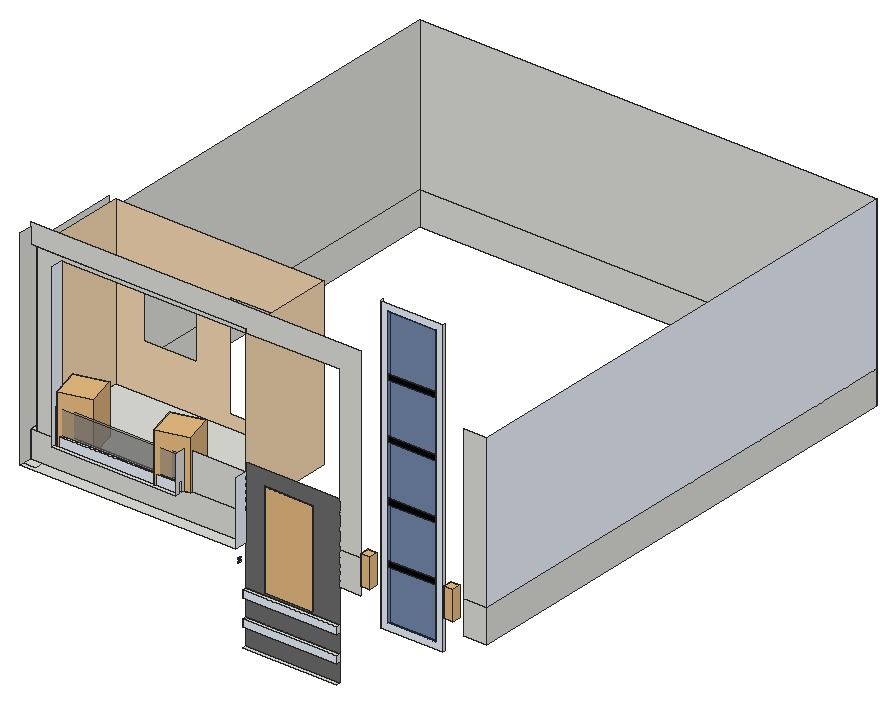
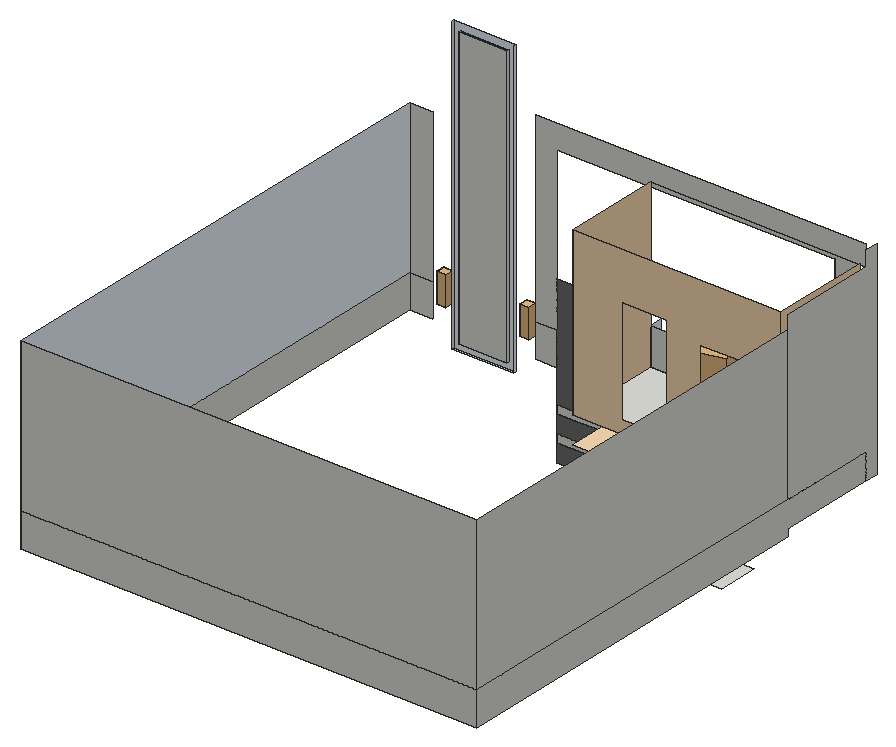
# SketchUp Ruby script. Lengths in inches.
U = 1.inch
M = Sketchup.active_model
def pt(a) = Geom::Point3d.new(a.map { |v| v * U })
def face(e, loops, mat)
  f = e.add_face(loops[0].map { |a| pt(a) })
  loops[1..].each { |l| e.add_face(l.map { |a| pt(a) }).erase! }
  f.material = f.back_material = mat if mat
  f
end
# faces: each face lists its corners as indices into pts; further lists are holes
def faces(e, pts, list, mat = nil) = list.each { |f| face(e, (f[0].is_a?(Array) ? f : [f]).map { |l| l.map { |i| pts[i] } }, mat) }
# xy, xz, yz: faces in a plane at the given z, y or x. An outline is a flat list of corners, or four numbers for a rectangle; further outlines are holes
def ring(l) = l.size == 4 ? [[l[0], l[1]], [l[2], l[1]], [l[2], l[3]], [l[0], l[3]]] : l.each_slice(2).to_a
def flat(e, list, mat, &to3) = list.each { |f| face(e, (f[0].is_a?(Array) ? f : [f]).map { |l| ring(l).map { |u, v| to3.(u, v) } }, mat) }
def xy(e, z, list, mat = nil) = flat(e, list, mat) { |x, y| [x, y, z] }
def xz(e, y, list, mat = nil) = flat(e, list, mat) { |x, z| [x, y, z] }
def yz(e, x, list, mat = nil) = flat(e, list, mat) { |y, z| [x, y, z] }
def lines(e, pts, list) = list.each { |a, b| e.add_line(pt(pts[a]), pt(pts[b])) }
# prism: a flat outline (further loops are holes) pulled along v
def prism(e, loops, v, mat = nil)
  f = face(e, loops, mat); d = Geom::Vector3d.new(v.map { |x| x * U })
  f.pushpull(f.normal.samedirection?(d) ? d.length : -d.length)
end
def box(e, o, s, mat = nil) = prism(e, [[o, [o[0] + s[0], o[1], o[2]], [o[0] + s[0], o[1] + s[1], o[2]], [o[0], o[1] + s[1], o[2]]]], [0, 0, s[2]], mat)
def at(x, y, z, deg = 0) = Geom::Transformation.translation(pt([x, y, z])) * Geom::Transformation.rotation(ORIGIN, Z_AXIS, deg.degrees)
def axes(o, x, y, z) = Geom::Transformation.new([*x, 0, *y, 0, *z, 0, *pt(o).to_a, 1])
def part(name) = M.definitions.add(name)
# library, detail: a bought-in or finely detailed component or shape, given as its bounding box
def library(name, o, s) = part(name).tap { |d| box(d.entities, o, s) }
def detail(e, o, s) = box(e.add_group.entities, o, s)
def put(e, d, t, mat = nil) = e.add_instance(d, t).tap { |i| i.material = mat if mat }
def group(e, t, mat = nil) = e.add_group.tap { |g| g.transformation = t; g.material = mat if mat }.entities
root = M.entities
M.materials.add("Generic").color = [111, 111, 111]
M.materials.add("Generic\#2").color = [253, 222, 182]
M.materials.add("Generic\#4").color = [238, 245, 255]
M.materials.add("Generic\#5").color = [7, 6, 6]
M.materials.add("Material \#1").color = [140, 140, 140]
M.materials.add("[Translucent Glass Blue]").color = [12, 53, 127]
M.materials["[Translucent Glass Blue]"].alpha = 0.5
M.materials.add("[Translucent Glass Gray]").color = [128, 128, 128]
M.materials["[Translucent Glass Gray]"].alpha = 0.5
c1 = library("3DGeom~14_Defintion",[-102.17,352.37,-727.27],[204.35,204.35,1000])
c2 = library("3DGeom~1_Defintion",[-60.87,347.29,-704.08],[121.74,121.75,1000])
c3 = library("adesivo+parede",[5.91,-0.05,0.37],[0.07,38.39,75.21])
c4 = library("Lamp Wall Outdoor 94-02",[-1.89,-4.65,-3.17],[3.78,4.65,6.35])
c5 = library("Group12\#2",[-37.1,-59.89,0],[61.11,59.71,94.13])
xy(root,52.376,[[169.979,34.653,243.692,37.591]])
xy(root,53.382,[[128.435,116.314,128.381,116.332,128.4375,116.329],[128.435,116.314,128.4375,116.329,128.489,116.329],[128.435,116.314,128.489,116.329,128.492,116.314],[128.492,116.314,128.489,116.329,128.537,116.346],[128.492,116.314,128.537,116.346,128.545,116.332],
  [128.4375,116.329,128.381,116.332,128.389,116.346],[128.381,116.332,128.337,116.367,128.389,116.346],[128.545,116.332,128.537,116.346,128.576,116.377],[128.545,116.332,128.576,116.377,128.589,116.367],[128.389,116.346,128.337,116.367,128.35,116.377],
  [128.337,116.367,128.309,116.413,128.35,116.377],[128.589,116.367,128.576,116.377,128.602,116.418],[128.589,116.367,128.602,116.418,128.617,116.413],[128.35,116.377,128.309,116.413,128.324,116.418],[128.309,116.413,128.299,116.465,128.324,116.418],
  [128.617,116.413,128.602,116.418,128.611,116.465],[128.617,116.413,128.611,116.465,128.627,116.465],[128.324,116.418,128.299,116.465,128.315,116.465],[128.299,116.465,128.309,116.518,128.315,116.465],[128.315,116.465,128.309,116.518,128.324,116.513],
  [128.611,116.465,128.602,116.513,128.627,116.465],[128.627,116.465,128.602,116.513,128.617,116.518],[128.324,116.513,128.309,116.518,128.337,116.564],[128.324,116.513,128.337,116.564,128.35,116.554],[128.602,116.513,128.576,116.554,128.617,116.518],
  [128.617,116.518,128.576,116.554,128.589,116.564],[128.35,116.554,128.337,116.564,128.381,116.598],[128.35,116.554,128.381,116.598,128.389,116.585],[128.576,116.554,128.537,116.585,128.589,116.564],[128.589,116.564,128.537,116.585,128.545,116.598],
  [128.389,116.585,128.381,116.598,128.435,116.616],[128.389,116.585,128.435,116.616,128.4375,116.601],[128.537,116.585,128.489,116.601,128.545,116.598],[128.545,116.598,128.489,116.601,128.492,116.616],[128.4375,116.601,128.435,116.616,128.492,116.616],
  [128.4375,116.601,128.492,116.616,128.489,116.601]],"Material \#1")
xy(root,53.397,[[128.435,116.314,128.389,116.346,128.381,116.332],[128.435,116.314,128.4375,116.329,128.389,116.346],[128.435,116.314,128.492,116.314,128.4375,116.329],[128.492,116.314,128.489,116.329,128.4375,116.329],[128.492,116.314,128.545,116.332,128.489,116.329],
  [128.489,116.329,128.545,116.332,128.537,116.346],[128.381,116.332,128.35,116.377,128.337,116.367],[128.381,116.332,128.389,116.346,128.35,116.377],[128.545,116.332,128.589,116.367,128.537,116.346],[128.537,116.346,128.589,116.367,128.576,116.377],
  [128.337,116.367,128.324,116.418,128.309,116.413],[128.337,116.367,128.35,116.377,128.324,116.418],[128.589,116.367,128.617,116.413,128.576,116.377],[128.576,116.377,128.617,116.413,128.602,116.418],[128.309,116.413,128.315,116.465,128.299,116.465],
  [128.309,116.413,128.324,116.418,128.315,116.465],[128.617,116.413,128.627,116.465,128.602,116.418],[128.602,116.418,128.627,116.465,128.611,116.465],[128.299,116.465,128.315,116.465,128.324,116.513],[128.299,116.465,128.324,116.513,128.309,116.518],
  [128.611,116.465,128.617,116.518,128.602,116.513],[128.611,116.465,128.627,116.465,128.617,116.518],[128.324,116.513,128.35,116.554,128.309,116.518],[128.602,116.513,128.589,116.564,128.576,116.554],[128.602,116.513,128.617,116.518,128.589,116.564],
  [128.309,116.518,128.35,116.554,128.337,116.564],[128.35,116.554,128.389,116.585,128.337,116.564],[128.576,116.554,128.545,116.598,128.537,116.585],[128.576,116.554,128.589,116.564,128.545,116.598],[128.337,116.564,128.389,116.585,128.381,116.598],
  [128.389,116.585,128.4375,116.601,128.381,116.598],[128.537,116.585,128.492,116.616,128.489,116.601],[128.537,116.585,128.545,116.598,128.492,116.616],[128.381,116.598,128.4375,116.601,128.435,116.616],[128.4375,116.601,128.489,116.601,128.435,116.616],
  [128.489,116.601,128.492,116.616,128.435,116.616]],"Material \#1")
xy(root,67.001,[[169.979,34.653,243.692,37.591]])
xy(root,72.939,[[169.979,34.653,243.692,37.591]])
xy(root,84.746,[[128.435,116.314,128.381,116.332,128.389,116.346],[128.435,116.314,128.389,116.346,128.4375,116.329],[128.435,116.314,128.4375,116.329,128.492,116.314],[128.492,116.314,128.4375,116.329,128.489,116.329],[128.492,116.314,128.489,116.329,128.545,116.332],
  [128.489,116.329,128.537,116.346,128.545,116.332],[128.381,116.332,128.337,116.367,128.35,116.377],[128.381,116.332,128.35,116.377,128.389,116.346],[128.545,116.332,128.537,116.346,128.589,116.367],[128.537,116.346,128.576,116.377,128.589,116.367],
  [128.337,116.367,128.309,116.413,128.324,116.418],[128.337,116.367,128.324,116.418,128.35,116.377],[128.589,116.367,128.576,116.377,128.617,116.413],[128.576,116.377,128.602,116.418,128.617,116.413],[128.309,116.413,128.299,116.465,128.315,116.465],
  [128.309,116.413,128.315,116.465,128.324,116.418],[128.617,116.413,128.602,116.418,128.627,116.465],[128.602,116.418,128.611,116.465,128.627,116.465],[128.299,116.465,128.309,116.518,128.324,116.513],[128.299,116.465,128.324,116.513,128.315,116.465],
  [128.611,116.465,128.602,116.513,128.617,116.518],[128.611,116.465,128.617,116.518,128.627,116.465],[128.324,116.513,128.309,116.518,128.35,116.554],[128.602,116.513,128.576,116.554,128.589,116.564],[128.602,116.513,128.589,116.564,128.617,116.518],
  [128.309,116.518,128.337,116.564,128.35,116.554],[128.35,116.554,128.337,116.564,128.389,116.585],[128.576,116.554,128.537,116.585,128.545,116.598],[128.576,116.554,128.545,116.598,128.589,116.564],[128.337,116.564,128.381,116.598,128.389,116.585],
  [128.389,116.585,128.381,116.598,128.4375,116.601],[128.537,116.585,128.489,116.601,128.492,116.616],[128.537,116.585,128.492,116.616,128.545,116.598],[128.381,116.598,128.435,116.616,128.4375,116.601],[128.4375,116.601,128.435,116.616,128.489,116.601],
  [128.489,116.601,128.435,116.616,128.492,116.616]],"Material \#1")
xy(root,84.762,[[128.435,116.314,128.4375,116.329,128.381,116.332],[128.435,116.314,128.489,116.329,128.4375,116.329],[128.435,116.314,128.492,116.314,128.489,116.329],[128.492,116.314,128.537,116.346,128.489,116.329],[128.492,116.314,128.545,116.332,128.537,116.346],
  [128.4375,116.329,128.389,116.346,128.381,116.332],[128.381,116.332,128.389,116.346,128.337,116.367],[128.545,116.332,128.576,116.377,128.537,116.346],[128.545,116.332,128.589,116.367,128.576,116.377],[128.389,116.346,128.35,116.377,128.337,116.367],
  [128.337,116.367,128.35,116.377,128.309,116.413],[128.589,116.367,128.602,116.418,128.576,116.377],[128.589,116.367,128.617,116.413,128.602,116.418],[128.35,116.377,128.324,116.418,128.309,116.413],[128.309,116.413,128.324,116.418,128.299,116.465],
  [128.617,116.413,128.611,116.465,128.602,116.418],[128.617,116.413,128.627,116.465,128.611,116.465],[128.324,116.418,128.315,116.465,128.299,116.465],[128.299,116.465,128.315,116.465,128.309,116.518],[128.315,116.465,128.324,116.513,128.309,116.518],
  [128.611,116.465,128.627,116.465,128.602,116.513],[128.627,116.465,128.617,116.518,128.602,116.513],[128.324,116.513,128.337,116.564,128.309,116.518],[128.324,116.513,128.35,116.554,128.337,116.564],[128.602,116.513,128.617,116.518,128.576,116.554],
  [128.617,116.518,128.589,116.564,128.576,116.554],[128.35,116.554,128.381,116.598,128.337,116.564],[128.35,116.554,128.389,116.585,128.381,116.598],[128.576,116.554,128.589,116.564,128.537,116.585],[128.589,116.564,128.545,116.598,128.537,116.585],
  [128.389,116.585,128.435,116.616,128.381,116.598],[128.389,116.585,128.4375,116.601,128.435,116.616],[128.537,116.585,128.545,116.598,128.489,116.601],[128.545,116.598,128.492,116.616,128.489,116.601],[128.4375,116.601,128.492,116.616,128.435,116.616],
  [128.4375,116.601,128.489,116.601,128.492,116.616]],"Material \#1")
xy(root,87.564,[[169.979,34.653,243.692,37.591]])
xy(root,87.784,[[27.056,114.716,68.556,146.403]])
xy(root,88.236,[[128.435,116.314,128.381,116.332,128.4375,116.329],[128.435,116.314,128.4375,116.329,128.489,116.329],[128.435,116.314,128.489,116.329,128.492,116.314],[128.492,116.314,128.489,116.329,128.537,116.346],[128.492,116.314,128.537,116.346,128.545,116.332],
  [128.4375,116.329,128.381,116.332,128.389,116.346],[128.381,116.332,128.337,116.367,128.389,116.346],[128.545,116.332,128.537,116.346,128.576,116.377],[128.545,116.332,128.576,116.377,128.589,116.367],[128.389,116.346,128.337,116.367,128.35,116.377],
  [128.337,116.367,128.309,116.413,128.35,116.377],[128.589,116.367,128.576,116.377,128.602,116.418],[128.589,116.367,128.602,116.418,128.617,116.413],[128.35,116.377,128.309,116.413,128.324,116.418],[128.309,116.413,128.299,116.465,128.324,116.418],
  [128.617,116.413,128.602,116.418,128.611,116.465],[128.617,116.413,128.611,116.465,128.627,116.465],[128.324,116.418,128.299,116.465,128.315,116.465],[128.299,116.465,128.309,116.518,128.315,116.465],[128.315,116.465,128.309,116.518,128.324,116.513],
  [128.611,116.465,128.602,116.513,128.627,116.465],[128.627,116.465,128.602,116.513,128.617,116.518],[128.324,116.513,128.309,116.518,128.337,116.564],[128.324,116.513,128.337,116.564,128.35,116.554],[128.602,116.513,128.576,116.554,128.617,116.518],
  [128.617,116.518,128.576,116.554,128.589,116.564],[128.35,116.554,128.337,116.564,128.381,116.598],[128.35,116.554,128.381,116.598,128.389,116.585],[128.576,116.554,128.537,116.585,128.589,116.564],[128.589,116.564,128.537,116.585,128.545,116.598],
  [128.389,116.585,128.381,116.598,128.435,116.616],[128.389,116.585,128.435,116.616,128.4375,116.601],[128.537,116.585,128.489,116.601,128.545,116.598],[128.545,116.598,128.489,116.601,128.492,116.616],[128.4375,116.601,128.435,116.616,128.492,116.616],
  [128.4375,116.601,128.492,116.616,128.489,116.601]],"Material \#1")
xy(root,88.251,[[128.435,116.314,128.389,116.346,128.381,116.332],[128.435,116.314,128.4375,116.329,128.389,116.346],[128.435,116.314,128.492,116.314,128.4375,116.329],[128.492,116.314,128.489,116.329,128.4375,116.329],[128.492,116.314,128.545,116.332,128.489,116.329],
  [128.489,116.329,128.545,116.332,128.537,116.346],[128.381,116.332,128.35,116.377,128.337,116.367],[128.381,116.332,128.389,116.346,128.35,116.377],[128.545,116.332,128.589,116.367,128.537,116.346],[128.537,116.346,128.589,116.367,128.576,116.377],
  [128.337,116.367,128.324,116.418,128.309,116.413],[128.337,116.367,128.35,116.377,128.324,116.418],[128.589,116.367,128.617,116.413,128.576,116.377],[128.576,116.377,128.617,116.413,128.602,116.418],[128.309,116.413,128.315,116.465,128.299,116.465],
  [128.309,116.413,128.324,116.418,128.315,116.465],[128.617,116.413,128.627,116.465,128.602,116.418],[128.602,116.418,128.627,116.465,128.611,116.465],[128.299,116.465,128.315,116.465,128.324,116.513],[128.299,116.465,128.324,116.513,128.309,116.518],
  [128.611,116.465,128.617,116.518,128.602,116.513],[128.611,116.465,128.627,116.465,128.617,116.518],[128.324,116.513,128.35,116.554,128.309,116.518],[128.602,116.513,128.589,116.564,128.576,116.554],[128.602,116.513,128.617,116.518,128.589,116.564],
  [128.309,116.518,128.35,116.554,128.337,116.564],[128.35,116.554,128.389,116.585,128.337,116.564],[128.576,116.554,128.545,116.598,128.537,116.585],[128.576,116.554,128.589,116.564,128.545,116.598],[128.337,116.564,128.389,116.585,128.381,116.598],
  [128.389,116.585,128.4375,116.601,128.381,116.598],[128.537,116.585,128.492,116.616,128.489,116.601],[128.537,116.585,128.545,116.598,128.492,116.616],[128.381,116.598,128.4375,116.601,128.435,116.616],[128.4375,116.601,128.489,116.601,128.435,116.616],
  [128.489,116.601,128.492,116.616,128.435,116.616]],"Material \#1")
xy(root,93.501,[[169.979,34.653,243.692,37.591]])
xy(root,95.774,[[95.002,114.716,130.44,133.091]])
xy(root,103.872,[[278.093,35.716,326.77,37.591]])
xy(root,109.492,[[283.712,35.716,321.15,37.591]])
xy(root,125.3125,[[0,27.716,0,30.841,9.75,30.841,9.75,37.591,169.979,37.591,169.979,27.716],[0,30.841,9.75,37.591]])
xy(root,125.3125,[[9.75,37.591,169.979,114.716]],"Generic\#2")
xy(root,146.375,[[24.805,27.716,122.632,30.759],[24.805,34.071,122.632,37.591],[0,37.591,5.4375,114.716],[5.4375,37.591,169.979,114.716]])
xy(root,154,[[[24.805,30.759,122.632,34.071],[25.395,31.35,122.041,33.481]]])
xz(root,30.759,[[24.805,146.375,122.632,154]],"Generic\#4")
xz(root,31.35,[[25.395,154,122.041,173.3125]],"[Translucent Glass Gray]")
xz(root,33.481,[[25.395,154,122.041,173.3125]],"[Translucent Glass Gray]")
xz(root,34.071,[[24.805,146.375,122.632,154]])
xz(root,34.653,[[169.979,67.001,243.692,72.939],[169.979,87.564,243.692,93.501]],"Generic\#4")
xz(root,35.716,[[[278.093,103.872,326.77,335.362],[283.712,109.492,321.15,329.742]]],"Generic\#4")
xz(root,37.591,[[169.979,67.001,243.692,72.939],[169.979,87.564,243.692,93.501],[283.712,109.492,321.15,329.742],[243.692,120,260.974,146.375],[342.12,120,360,146.375],
  [0,125.3125,169.979,146.375],[243.692,146.375,243.692,273.875,169.979,273.875,169.979,276.8125,0,276.8125,0,292.75,260.974,292.75,260.974,146.375],[5.4375,146.375,5.4375,276.8125,169.979,276.8125,169.979,273.875,24.805,273.875,24.805,146.375],[122.632,146.375,169.979,175.6875],[342.12,146.375,360,266.375]])
xz(root,37.591,[[169.979,52.376,243.692,67.001],[169.979,72.939,243.692,87.564],[169.979,93.501,243.692,182.626]],"Generic")
xz(root,114.716,[[[5.4375,146.375,169.979,276.8125],[95.815,156.586,131.252,239.461],[27.868,184.097,69.368,231.472]]],"Generic\#2")
xz(root,115.852,[[100.828,55.493,100.819,55.494,100.828,55.62],[100.828,55.493,100.828,55.62,100.838,55.618],[101.957,55.493,101.948,55.618,101.967,55.494],[101.967,55.494,101.948,55.618,101.957,55.62],[101.393,55.544,101.359,55.548,101.393,55.556],
  [101.393,55.544,101.393,55.556,101.425,55.559],[101.393,55.544,101.425,55.559,101.427,55.548],[101.359,55.548,101.326,55.558,101.36,55.559],[101.359,55.548,101.36,55.559,101.393,55.556],[101.427,55.548,101.425,55.559,101.456,55.569],
  [101.427,55.548,101.456,55.569,101.459,55.558],[101.326,55.558,101.297,55.575,101.33,55.569],[101.326,55.558,101.33,55.569,101.36,55.559],[101.459,55.558,101.456,55.569,101.484,55.585],[101.459,55.558,101.484,55.585,101.489,55.575],
  [101.33,55.569,101.297,55.575,101.302,55.585],[101.297,55.575,101.27,55.597,101.302,55.585],[101.489,55.575,101.484,55.585,101.509,55.606],[101.489,55.575,101.509,55.606,101.516,55.597],[101.302,55.585,101.27,55.597,101.276,55.606],
  [101.27,55.597,101.247,55.624,101.276,55.606],[101.516,55.597,101.509,55.606,101.531,55.632],[101.516,55.597,101.531,55.632,101.539,55.624],[101.276,55.606,101.247,55.624,101.255,55.632],[100.838,55.618,100.828,55.62,100.855,55.734],
  [100.838,55.618,100.855,55.734,100.864,55.73],[101.948,55.618,101.921,55.73,101.957,55.62],[101.957,55.62,101.921,55.73,101.931,55.734],[101.247,55.624,101.228,55.656,101.255,55.632],[101.539,55.624,101.531,55.632,101.549,55.662],
  [101.539,55.624,101.549,55.662,101.557,55.656],[101.255,55.632,101.228,55.656,101.237,55.662],[101.228,55.656,101.214,55.691,101.237,55.662],[101.557,55.656,101.549,55.662,101.562,55.695],[101.557,55.656,101.562,55.695,101.571,55.691],
  [101.237,55.662,101.214,55.691,101.223,55.695],[101.214,55.691,101.205,55.729,101.223,55.695],[101.571,55.691,101.562,55.695,101.571,55.731],[101.571,55.691,101.571,55.731,101.58,55.729],[101.223,55.695,101.205,55.729,101.215,55.731],
  [101.205,55.729,101.202,55.78,101.215,55.731],[101.58,55.729,101.571,55.731,101.574,55.769],[101.58,55.729,101.574,55.769,101.583,55.769],[100.864,55.73,100.855,55.734,100.897,55.84],[100.864,55.73,100.897,55.84,100.906,55.834],
  [101.921,55.73,101.88,55.834,101.931,55.734],[101.215,55.731,101.202,55.78,101.212,55.78],[101.931,55.734,101.88,55.834,101.888,55.84],[101.574,55.769,101.571,55.807,101.583,55.769],[101.583,55.769,101.571,55.807,101.58,55.81],
  [101.202,55.78,101.205,55.81,101.212,55.78],[101.212,55.78,101.205,55.81,101.215,55.807],[101.215,55.807,101.205,55.81,101.214,55.848],[101.215,55.807,101.214,55.848,101.223,55.844],[101.571,55.807,101.562,55.844,101.58,55.81],
  [101.58,55.81,101.562,55.844,101.571,55.848],[100.906,55.834,100.897,55.84,100.956,55.938],[100.906,55.834,100.956,55.938,100.964,55.93],[101.88,55.834,101.824,55.927,101.888,55.84],[101.888,55.84,101.824,55.927,101.832,55.934],
  [101.223,55.844,101.214,55.848,101.228,55.883],[101.223,55.844,101.228,55.883,101.237,55.877],[101.562,55.844,101.549,55.877,101.571,55.848],[101.571,55.848,101.549,55.877,101.557,55.883],[101.237,55.877,101.228,55.883,101.247,55.914],
  [101.237,55.877,101.247,55.914,101.255,55.907],[101.549,55.877,101.531,55.907,101.557,55.883],[101.557,55.883,101.531,55.907,101.539,55.914],[101.255,55.907,101.247,55.914,101.27,55.941],[101.255,55.907,101.27,55.941,101.276,55.932],
  [101.531,55.907,101.509,55.932,101.539,55.914],[101.539,55.914,101.509,55.932,101.516,55.941],[101.824,55.927,101.756,56.007,101.832,55.934],[100.964,55.93,100.956,55.938,101.023,56.016],[100.964,55.93,101.023,56.016,101.03,56.007],
  [101.276,55.932,101.27,55.941,101.297,55.964],[101.276,55.932,101.297,55.964,101.302,55.953],[101.509,55.932,101.484,55.953,101.516,55.941],[101.832,55.934,101.756,56.007,101.762,56.016],[101.516,55.941,101.484,55.953,101.489,55.964],
  [101.302,55.953,101.297,55.964,101.326,55.98],[101.302,55.953,101.326,55.98,101.33,55.969],[101.484,55.953,101.456,55.969,101.489,55.964],[101.489,55.964,101.456,55.969,101.459,55.98],[101.33,55.969,101.326,55.98,101.359,55.991],
  [101.33,55.969,101.359,55.991,101.36,55.979],[101.456,55.969,101.425,55.979,101.459,55.98],[101.36,55.979,101.359,55.991,101.393,55.994],[101.36,55.979,101.393,55.994,101.393,55.983],[101.425,55.979,101.393,55.983,101.427,55.991],
  [101.425,55.979,101.427,55.991,101.459,55.98],[101.393,55.983,101.393,55.994,101.427,55.991],[101.03,56.007,101.023,56.016,101.103,56.083],[101.03,56.007,101.103,56.083,101.108,56.073],[101.756,56.007,101.677,56.073,101.762,56.016],
  [101.762,56.016,101.677,56.073,101.682,56.083],[101.108,56.073,101.103,56.083,101.193,56.133],[101.108,56.073,101.193,56.133,101.196,56.122],[101.677,56.073,101.589,56.122,101.682,56.083],[101.682,56.083,101.589,56.122,101.593,56.133],
  [101.196,56.122,101.193,56.133,101.29,56.165],[101.196,56.122,101.29,56.165,101.291,56.153],[101.589,56.122,101.494,56.153,101.593,56.133],[101.593,56.133,101.494,56.153,101.496,56.165],[101.291,56.153,101.29,56.165,101.393,56.176],
  [101.291,56.153,101.393,56.176,101.393,56.164],[101.494,56.153,101.393,56.164,101.496,56.165],[101.393,56.164,101.393,56.176,101.496,56.165]],"Material \#1")
xz(root,117.632,[[100.828,55.493,100.828,55.62,100.819,55.494],[100.828,55.493,100.838,55.618,100.828,55.62],[101.957,55.493,101.967,55.494,101.948,55.618],[101.967,55.494,101.957,55.62,101.948,55.618],[101.393,55.544,101.393,55.556,101.359,55.548],
  [101.393,55.544,101.425,55.559,101.393,55.556],[101.393,55.544,101.427,55.548,101.425,55.559],[101.359,55.548,101.36,55.559,101.326,55.558],[101.359,55.548,101.393,55.556,101.36,55.559],[101.427,55.548,101.456,55.569,101.425,55.559],
  [101.427,55.548,101.459,55.558,101.456,55.569],[101.326,55.558,101.33,55.569,101.297,55.575],[101.326,55.558,101.36,55.559,101.33,55.569],[101.459,55.558,101.484,55.585,101.456,55.569],[101.459,55.558,101.489,55.575,101.484,55.585],
  [101.33,55.569,101.302,55.585,101.297,55.575],[101.297,55.575,101.302,55.585,101.27,55.597],[101.489,55.575,101.509,55.606,101.484,55.585],[101.489,55.575,101.516,55.597,101.509,55.606],[101.302,55.585,101.276,55.606,101.27,55.597],
  [101.27,55.597,101.276,55.606,101.247,55.624],[101.516,55.597,101.531,55.632,101.509,55.606],[101.516,55.597,101.539,55.624,101.531,55.632],[101.276,55.606,101.255,55.632,101.247,55.624],[100.838,55.618,100.855,55.734,100.828,55.62],
  [100.838,55.618,100.864,55.73,100.855,55.734],[101.948,55.618,101.957,55.62,101.921,55.73],[101.957,55.62,101.931,55.734,101.921,55.73],[101.247,55.624,101.255,55.632,101.228,55.656],[101.539,55.624,101.549,55.662,101.531,55.632],
  [101.539,55.624,101.557,55.656,101.549,55.662],[101.255,55.632,101.237,55.662,101.228,55.656],[101.228,55.656,101.237,55.662,101.214,55.691],[101.557,55.656,101.562,55.695,101.549,55.662],[101.557,55.656,101.571,55.691,101.562,55.695],
  [101.237,55.662,101.223,55.695,101.214,55.691],[101.214,55.691,101.223,55.695,101.205,55.729],[101.571,55.691,101.571,55.731,101.562,55.695],[101.571,55.691,101.58,55.729,101.571,55.731],[101.223,55.695,101.215,55.731,101.205,55.729],
  [101.205,55.729,101.215,55.731,101.202,55.78],[101.58,55.729,101.574,55.769,101.571,55.731],[101.58,55.729,101.583,55.769,101.574,55.769],[100.864,55.73,100.897,55.84,100.855,55.734],[100.864,55.73,100.906,55.834,100.897,55.84],
  [101.921,55.73,101.931,55.734,101.88,55.834],[101.215,55.731,101.212,55.78,101.202,55.78],[101.931,55.734,101.888,55.84,101.88,55.834],[101.574,55.769,101.583,55.769,101.571,55.807],[101.583,55.769,101.58,55.81,101.571,55.807],
  [101.202,55.78,101.212,55.78,101.205,55.81],[101.212,55.78,101.215,55.807,101.205,55.81],[101.215,55.807,101.214,55.848,101.205,55.81],[101.215,55.807,101.223,55.844,101.214,55.848],[101.571,55.807,101.58,55.81,101.562,55.844],
  [101.58,55.81,101.571,55.848,101.562,55.844],[100.906,55.834,100.956,55.938,100.897,55.84],[100.906,55.834,100.964,55.93,100.956,55.938],[101.88,55.834,101.888,55.84,101.824,55.927],[101.888,55.84,101.832,55.934,101.824,55.927],
  [101.223,55.844,101.228,55.883,101.214,55.848],[101.223,55.844,101.237,55.877,101.228,55.883],[101.562,55.844,101.571,55.848,101.549,55.877],[101.571,55.848,101.557,55.883,101.549,55.877],[101.237,55.877,101.247,55.914,101.228,55.883],
  [101.237,55.877,101.255,55.907,101.247,55.914],[101.549,55.877,101.557,55.883,101.531,55.907],[101.557,55.883,101.539,55.914,101.531,55.907],[101.255,55.907,101.27,55.941,101.247,55.914],[101.255,55.907,101.276,55.932,101.27,55.941],
  [101.531,55.907,101.539,55.914,101.509,55.932],[101.539,55.914,101.516,55.941,101.509,55.932],[101.824,55.927,101.832,55.934,101.756,56.007],[100.964,55.93,101.023,56.016,100.956,55.938],[100.964,55.93,101.03,56.007,101.023,56.016],
  [101.276,55.932,101.297,55.964,101.27,55.941],[101.276,55.932,101.302,55.953,101.297,55.964],[101.509,55.932,101.516,55.941,101.484,55.953],[101.832,55.934,101.762,56.016,101.756,56.007],[101.516,55.941,101.489,55.964,101.484,55.953],
  [101.302,55.953,101.326,55.98,101.297,55.964],[101.302,55.953,101.33,55.969,101.326,55.98],[101.484,55.953,101.489,55.964,101.456,55.969],[101.489,55.964,101.459,55.98,101.456,55.969],[101.33,55.969,101.359,55.991,101.326,55.98],
  [101.33,55.969,101.36,55.979,101.359,55.991],[101.456,55.969,101.459,55.98,101.425,55.979],[101.36,55.979,101.393,55.994,101.359,55.991],[101.36,55.979,101.393,55.983,101.393,55.994],[101.425,55.979,101.427,55.991,101.393,55.983],
  [101.425,55.979,101.459,55.98,101.427,55.991],[101.393,55.983,101.427,55.991,101.393,55.994],[101.03,56.007,101.103,56.083,101.023,56.016],[101.03,56.007,101.108,56.073,101.103,56.083],[101.756,56.007,101.762,56.016,101.677,56.073],
  [101.762,56.016,101.682,56.083,101.677,56.073],[101.108,56.073,101.193,56.133,101.103,56.083],[101.108,56.073,101.196,56.122,101.193,56.133],[101.677,56.073,101.682,56.083,101.589,56.122],[101.682,56.083,101.593,56.133,101.589,56.122],
  [101.196,56.122,101.29,56.165,101.193,56.133],[101.196,56.122,101.291,56.153,101.29,56.165],[101.589,56.122,101.593,56.133,101.494,56.153],[101.593,56.133,101.496,56.165,101.494,56.153],[101.291,56.153,101.393,56.176,101.29,56.165],
  [101.291,56.153,101.393,56.164,101.393,56.176],[101.494,56.153,101.496,56.165,101.393,56.164],[101.393,56.164,101.496,56.165,101.393,56.176]],"Material \#1")
xz(root,421.591,[[0,120,360,146.375],[0,146.375,360,266.375]])
yz(root,0,[[114.716,120,114.716,125.3125,37.591,125.3125,37.591,146.375,421.591,146.375,421.591,120],[27.716,125.3125,27.716,288.8125,37.591,288.8125,37.591,276.8125,114.716,276.8125,114.716,146.375,37.591,146.375,37.591,125.3125],[114.716,146.375,421.591,266.375]])
yz(root,5.4375,[[37.591,146.375,114.716,276.8125]],"Generic\#2")
yz(root,24.805,[[27.716,146.375,30.759,146.375,30.759,154,34.071,154,34.071,146.375,37.591,146.375,37.591,273.875,27.716,273.875]],"Generic\#4")
yz(root,25.395,[[31.35,154,33.481,173.3125]])
yz(root,122.041,[[31.35,154,33.481,173.3125]])
yz(root,122.632,[[27.716,146.375,27.716,175.6875,37.591,175.6875,37.591,146.375,34.071,146.375,34.071,154,30.759,154,30.759,146.375]])
yz(root,169.979,[[34.653,67.001,37.591,72.939],[34.653,87.564,37.591,93.501]])
yz(root,169.979,[[37.591,146.375,114.716,276.8125]],"Generic\#2")
yz(root,169.979,[[27.716,125.3125,37.591,175.6875]],"Generic\#4")
yz(root,243.692,[[34.653,67.001,37.591,72.939],[34.653,87.564,37.591,93.501]])
yz(root,278.093,[[35.716,103.872,37.591,335.362]],"Generic\#4")
yz(root,283.712,[[35.716,109.492,37.591,329.742]])
yz(root,321.15,[[35.716,109.492,37.591,329.742]])
yz(root,326.77,[[35.716,103.872,37.591,335.362]])
yz(root,360,[[37.591,120,421.591,146.375]])
yz(root,360,[[37.591,146.375,421.591,266.375]],"Generic\#4")
p = [[101.415,115.851,55.671],[101.415,115.876,55.671],[101.428,115.882,55.646],[101.428,115.858,55.646],[101.448,115.882,55.656],[101.448,115.858,55.656],
  [101.415,117.632,55.671],[101.428,117.625,55.646],[101.428,117.601,55.646],[101.415,117.607,55.671],[101.448,117.625,55.656],[101.448,117.601,55.656],
  [101.343,115.849,55.818],[101.343,115.873,55.818],[101.404,115.873,55.694],[101.404,115.849,55.694],[101.442,115.873,55.72],[101.442,115.849,55.72],
  [101.454,115.851,55.698],[101.382,115.873,55.844],[101.382,115.849,55.844],[101.466,115.882,55.672],[101.466,115.858,55.672],[101.454,115.876,55.698],
  [101.343,117.634,55.818],[101.404,117.634,55.694],[101.404,117.61,55.694],[101.343,117.61,55.818],[101.466,117.625,55.672],[101.466,117.601,55.672],
  [101.454,117.632,55.698],[101.442,117.634,55.72],[101.442,117.61,55.72],[101.454,117.607,55.698],[101.382,117.634,55.844],[101.382,117.61,55.844],
  [101.332,115.851,55.841],[101.371,115.876,55.867],[101.371,115.851,55.867],[101.319,115.858,55.867],[101.319,115.882,55.867],[101.332,115.876,55.841],
  [101.319,117.625,55.867],[101.332,117.632,55.841],[101.332,117.607,55.841],[101.319,117.601,55.867],[101.371,117.632,55.867],[101.371,117.607,55.867],
  [101.358,115.858,55.893],[101.358,115.882,55.893],[101.337,115.882,55.883],[101.337,115.858,55.883],[101.358,117.625,55.893],[101.337,117.625,55.883],
  [101.337,117.601,55.883],[101.358,117.601,55.893]]
faces(root,p,[[0,1,2],[2,3,0],[3,2,4],[4,5,3],[6,7,8],[8,9,6],[7,10,11],[11,8,7],
  [12,13,14],[14,15,12],[15,14,1],[1,0,15],[16,17,18],[17,16,19],[19,20,17],[5,4,21],
  [21,22,5],[18,23,16],[22,21,23],[23,18,22],[24,25,26],[26,27,24],[25,6,9],[9,26,25],
  [10,28,29],[29,11,10],[30,31,32],[32,33,30],[31,34,35],[35,32,31],[28,30,33],[33,29,28],
  [13,12,36],[20,19,37],[37,38,20],[39,40,41],[41,36,39],[36,41,13],[42,43,44],[44,45,42],
  [43,24,27],[27,44,43],[34,46,47],[47,35,34],[48,49,50],[50,51,48],[51,50,40],[40,39,51],
  [38,37,49],[49,48,38],[52,53,54],[54,55,52],[53,42,45],[45,54,53],[46,52,55],[55,47,46]],"Material \#1")
put(root,c1,axes([101.39,117.36,51.625],[0.00289,0,0],[0,0,0.00341],[0,0.0027,0]),"Material \#1")
put(root,c2,axes([101.39,117.36,51.625],[0.00322,0,0],[0,0,0.0038],[0,0.00301,0]),"Material \#1")
put(root,c3,at(189.46,37.59,99.12,-90))
g1 = group(root,at(283.71,35.72,109.49),"Generic\#5")
xz(g1,0,[[0,39.74,37.4375,44.05],[0,83.79,37.4375,88.1],[0,127.84,37.4375,132.15],[0,171.89,37.4375,176.2]])
xz(g1,0,[[0,0,37.4375,39.74],[0,44.05,37.4375,83.79],[0,88.1,37.4375,127.84],[0,132.15,37.4375,171.89],[0,176.2,37.4375,220.25]],"[Translucent Glass Blue]")
put(root,c4,axes([269.82,37.59,143.1875],[1.9536,0,0],[0,1.48,0],[0,0,3.6112]),"Generic\#5")
put(root,c4,axes([335.13,37.59,143.1875],[1.9536,0,0],[0,1.48,0],[0,0,3.6112]),"Generic\#5")
put(root,c5,axes([34.81,58.04,146.375],[0.39603,0.10612,0],[-0.10612,0.39603,0],[0,0,0.41]))
put(root,c5,axes([111.56,58.04,146.375],[0.39603,0.10612,0],[-0.10612,0.39603,0],[0,0,0.41]))
